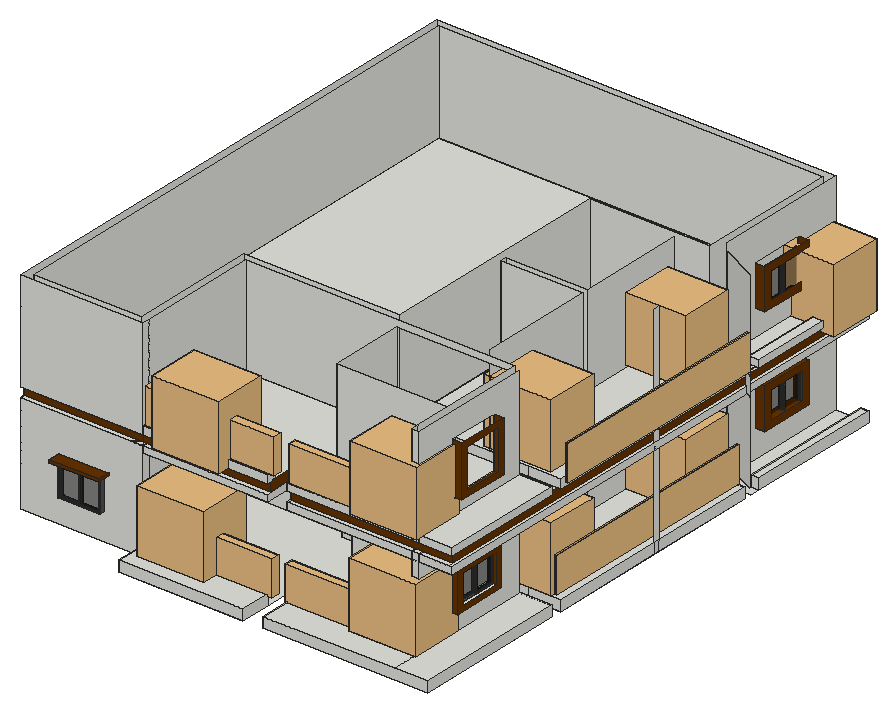
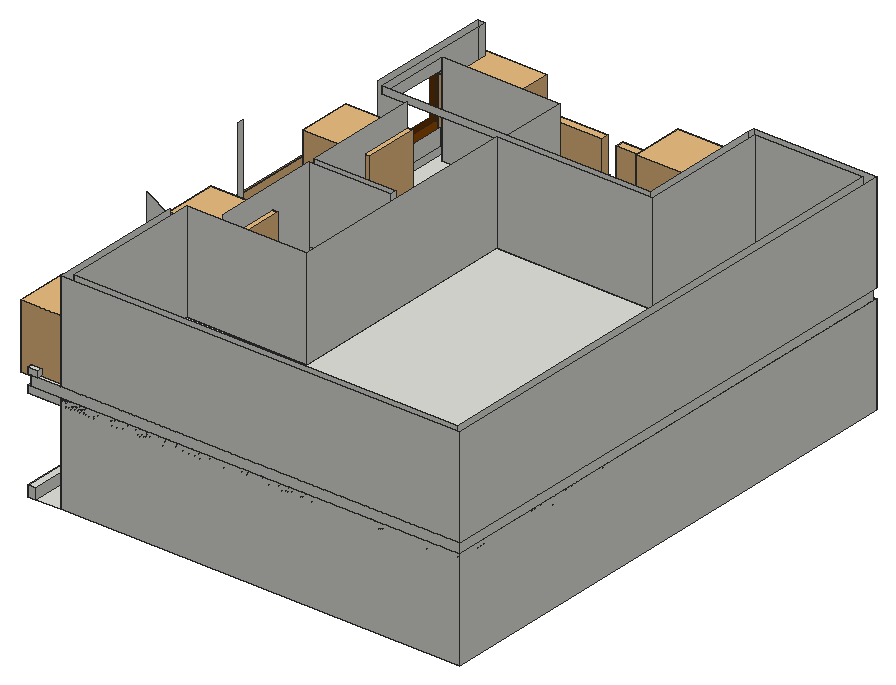
# SketchUp Ruby script. Lengths in inches.
U = 1.inch
M = Sketchup.active_model
def pt(a) = Geom::Point3d.new(a.map { |v| v * U })
def face(e, loops, mat)
  f = e.add_face(loops[0].map { |a| pt(a) })
  loops[1..].each { |l| e.add_face(l.map { |a| pt(a) }).erase! }
  f.material = f.back_material = mat if mat
  f
end
# faces: each face lists its corners as indices into pts; further lists are holes
def faces(e, pts, list, mat = nil) = list.each { |f| face(e, (f[0].is_a?(Array) ? f : [f]).map { |l| l.map { |i| pts[i] } }, mat) }
# xy, xz, yz: faces in a plane at the given z, y or x. An outline is a flat list of corners, or four numbers for a rectangle; further outlines are holes
def ring(l) = l.size == 4 ? [[l[0], l[1]], [l[2], l[1]], [l[2], l[3]], [l[0], l[3]]] : l.each_slice(2).to_a
def flat(e, list, mat, &to3) = list.each { |f| face(e, (f[0].is_a?(Array) ? f : [f]).map { |l| ring(l).map { |u, v| to3.(u, v) } }, mat) }
def xy(e, z, list, mat = nil) = flat(e, list, mat) { |x, y| [x, y, z] }
def xz(e, y, list, mat = nil) = flat(e, list, mat) { |x, z| [x, y, z] }
def yz(e, x, list, mat = nil) = flat(e, list, mat) { |y, z| [x, y, z] }
def lines(e, pts, list) = list.each { |a, b| e.add_line(pt(pts[a]), pt(pts[b])) }
# prism: a flat outline (further loops are holes) pulled along v
def prism(e, loops, v, mat = nil)
  f = face(e, loops, mat); d = Geom::Vector3d.new(v.map { |x| x * U })
  f.pushpull(f.normal.samedirection?(d) ? d.length : -d.length)
end
def box(e, o, s, mat = nil) = prism(e, [[o, [o[0] + s[0], o[1], o[2]], [o[0] + s[0], o[1] + s[1], o[2]], [o[0], o[1] + s[1], o[2]]]], [0, 0, s[2]], mat)
def at(x, y, z, deg = 0) = Geom::Transformation.translation(pt([x, y, z])) * Geom::Transformation.rotation(ORIGIN, Z_AXIS, deg.degrees)
def axes(o, x, y, z) = Geom::Transformation.new([*x, 0, *y, 0, *z, 0, *pt(o).to_a, 1])
def part(name) = M.definitions.add(name)
# library, detail: a bought-in or finely detailed component or shape, given as its bounding box
def library(name, o, s) = part(name).tap { |d| box(d.entities, o, s) }
def detail(e, o, s) = box(e.add_group.entities, o, s)
def put(e, d, t, mat = nil) = e.add_instance(d, t).tap { |i| i.material = mat if mat }
def group(e, t, mat = nil) = e.add_group.tap { |g| g.transformation = t; g.material = mat if mat }.entities
root = M.entities
M.materials.add("Glass_Tinted_Gray").color = [0, 0, 0]
M.materials["Glass_Tinted_Gray"].alpha = 0.125
M.materials.add("[0135_DarkGray]").color = [81, 81, 81]
M.materials.add("[Color C08]").color = [102, 51, 0]
M.materials.add("[Mirror 02]").color = [229, 229, 229]
M.materials.add("[Terrazzo Light Blue]").color = [196, 214, 227]
c1 = library("Round Planter with Plant",[-35.48,-39.77,0],[80.62,63.55,77.875])
c2 = library("Wagner Glass Railing",[9.08,102.375,1.53],[2.51,145.5,42.05])
c3 = part("PENTEK_RP Fineline 50S_Sliding_DoorCase_E1")
box(c3.entities,[0,0,0],[1.51,3.66,99.27],"[0135_DarkGray]")
c4 = part("PENTEK_RP Fineline 50S_SlidingDooe_Case_E2")
box(c4.entities,[0,0,0],[96.25,3.66,1.51],"[0135_DarkGray]")
c5 = part("pentek_RP Fineline 50S_SlidingDoor_Case")
put(c5.entities,c3,at(97.76,0,0))
put(c5.entities,c4,at(1.51,0,0))
put(c5.entities,c3,at(0,0,0))
put(c5.entities,c4,at(1.51,0,97.76))
c6 = part("PENTEK_RP Fineline 50S_SlidingDoor_GlazingBead_2")
box(c6.entities,[0,0,0],[0.56,0.59,94.39],"[0135_DarkGray]")
c7 = part("PENTEK_RP Fineline 50S_SlidingDoor_Glass")
box(c7.entities,[0,0,0],[46.58,0.16,94.39],"Glass_Tinted_Gray")
c8 = part("PENTEK_RP Fineline 50S_SlidingDoor_GlazingBead")
box(c8.entities,[0,0,0],[45.47,0.59,0.56],"[0135_DarkGray]")
c9 = part("PENTEK_RP Fineline 50S_SlidingDoor_Leaf_E1")
xy(c9.entities,0,[[0,0,0.93,1.97],[0.93,1.57,1.49,1.97]],"[0135_DarkGray]")
xy(c9.entities,96.25,[[0,0,0.93,0,0.93,1.57,1.49,1.57,1.49,1.97,0,1.97]],"[0135_DarkGray]")
xz(c9.entities,0,[[0,0,0.93,96.25]],"[0135_DarkGray]")
xz(c9.entities,1.57,[[0.93,0,1.49,95.32],[0.93,95.32,1.49,96.25]],"[0135_DarkGray]")
xz(c9.entities,1.97,[[0,0,1.49,96.25]],"[0135_DarkGray]")
yz(c9.entities,0,[[0,0,1.97,96.25]],"[0135_DarkGray]")
yz(c9.entities,0.93,[[0,0,1.57,0.93],[0,0.93,1.57,95.32],[0,95.32,1.57,96.25]],"[0135_DarkGray]")
yz(c9.entities,1.49,[[1.57,0,1.97,95.32],[1.57,95.32,1.97,96.25]],"[0135_DarkGray]")
c10 = part("PENTEK_RP Fineline 50S_SlidingDoor_Leaf_E2")
xy(c10.entities,0,[[0,0,0,1.57,0.56,1.57,0.56,1.97,46.02,1.97,46.02,1.57,46.58,1.57,46.58,0]],"[0135_DarkGray]")
xy(c10.entities,0.93,[[0,0,46.58,1.57]],"[0135_DarkGray]")
xy(c10.entities,1.49,[[0.56,1.57,46.02,1.97]],"[0135_DarkGray]")
xz(c10.entities,0,[[0,0,46.58,0.93]],"[0135_DarkGray]")
xz(c10.entities,1.57,[[0,0,0.56,0.93],[46.02,0,46.58,0.93],[0.56,0.93,46.02,1.49]],"[0135_DarkGray]")
xz(c10.entities,1.97,[[0.56,0,46.02,1.49]],"[0135_DarkGray]")
yz(c10.entities,0,[[0,0,1.57,0.93]],"[0135_DarkGray]")
yz(c10.entities,0.56,[[1.57,0,1.97,0.93],[1.57,0.93,1.97,1.49]],"[0135_DarkGray]")
yz(c10.entities,46.02,[[1.57,0,1.97,0.93],[1.57,0.93,1.97,1.49]],"[0135_DarkGray]")
yz(c10.entities,46.58,[[0,0,1.57,0.93]],"[0135_DarkGray]")
c11 = part("PENTEK_RP Fineline S_SlidingDoor_Leaf1")
put(c11.entities,c6,at(0.93,0,0.93))
put(c11.entities,c6,at(46.96,0,0.93))
put(c11.entities,c7,at(1.49,1.42,0.93))
put(c11.entities,c8,at(1.49,0,0.93))
put(c11.entities,c7,at(1.49,0.59,0.93),"[Terrazzo Light Blue]")
put(c11.entities,c9,at(0,0,0))
put(c11.entities,c9,axes([48.44,0,0],[-1,0,0],[0,1,0],[0,0,1]))
put(c11.entities,c10,axes([0.93,0,96.25],[1,0,0],[0,1,0],[0,0,-1]))
put(c11.entities,c10,at(0.93,0,0))
put(c11.entities,c8,at(1.49,0,94.77))
c12 = part("PENTEK_RP Fineline 50S_SlidingDoor_Leaf2")
put(c12.entities,c7,at(1.49,1.42,0.93))
put(c12.entities,c8,at(1.49,0,94.77))
put(c12.entities,c6,at(46.96,0,0.93))
put(c12.entities,c7,at(1.49,0.59,0.93),"[Mirror 02]")
put(c12.entities,c6,at(0.93,0,0.93))
put(c12.entities,c9,at(0,0,0))
put(c12.entities,c9,axes([48.44,0,0],[-1,0,0],[0,1,0],[0,0,1]))
put(c12.entities,c8,at(1.49,0,0.93))
put(c12.entities,c10,axes([0.93,0,96.25],[1,0,0],[0,1,0],[0,0,-1]))
put(c12.entities,c10,at(0.93,0,0))
c13 = part("PENTEK - Slimmest Steel Sliding Door / Window\#1")
put(c13.entities,c5,at(0,-1.88,-0.09))
put(c13.entities,c11,at(1.51,-2.27,1.42))
put(c13.entities,c12,at(49.32,-0.3,1.42))
c14 = part("Group\#9")
box(c14.entities,[0,0,0],[60.1875,3.0625,15.3125])
xy(root,264,[[200.56,155.07,350.31,191.22],[374.31,155.07,532.37,191.22],[532.37,155.07,562.5625,155.07,562.5625,162,572.25,162,572.25,341.375,533.0625,341.375,533.0625,191.22,532.37,191.22],[562.5625,155.07,572.25,162],[[53.0625,191.22,200.56,191.22,200.56,346.01,322.375,346.01,322.375,338.57,390.45,338.57,390.45,267.82,524.0625,267.82,524.0625,191.22,532.37,191.22,532.37,341.375,533.0625,341.375,533.0625,355.01,388.3125,355.01,388.3125,631.35,533.0625,631.35,533.0625,818.16,53.0625,818.16],[62.0625,200.22,62.0625,809.84,524.0625,809.84,524.0625,640.35,379.3125,640.35,379.3125,355.01,191.56,355.01,191.56,200.22]],
  [200.56,191.22,350.31,191.22,350.31,232.22,374.31,232.22,374.31,191.22,524.0625,191.22,524.0625,267.82,390.45,267.82,390.45,338.57,322.375,338.57,322.375,346.01,200.56,346.01],[532.37,191.22,533.0625,341.375],[62.0625,200.22,191.56,200.22,191.56,355.01,379.3125,355.01,379.3125,640.35,524.0625,640.35,524.0625,809.84,62.0625,809.84],[388.3125,355.01,572.25,631.35],[533.0625,641.54,572.25,641.54,572.25,653.47,562.82,653.47,562.82,818.16,533.0625,818.16]])
xy(root,276.5625,[[200.56,155.07,350.31,191.22],[374.31,155.07,532.37,191.22],[532.37,155.07,572.25,341.375],[388.3125,355.01,486.8125,495.28],[486.8125,355.01,572.25,355.01,572.25,631.35,486.8125,631.35,486.8125,502.74,388.3125,502.74,388.3125,495.28,486.8125,495.28],
  [388.3125,502.74,486.8125,631.35],[562.82,653.47,572.25,818.16]])
xy(root,298.54,[[533.0625,696.28,545.1875,761.47]],"[Color C08]")
xy(root,303.83,[[533.0625,234.02,545.1875,299.52]],"[Color C08]")
xy(root,306.6,[[533.0625,704.34,545.1875,753.42]],"[Color C08]")
xy(root,310.91,[[533.0625,241.1,545.1875,292.4375]])
xy(root,339.68,[[533.0625,704.34,545.1875,753.42]])
xy(root,346.18,[[533.0625,241.1,545.1875,292.4375]],"[Color C08]")
xy(root,347.73,[[533.0625,696.28,545.1875,761.47]],"[Color C08]")
xy(root,353.26,[[533.0625,234.02,545.1875,299.52]],"[Color C08]")
xy(root,375.8125,[[390.45,267.82,524.0625,267.82,524.0625,346.01,412.14,346.01,412.14,338.57,390.45,338.57],[322.375,338.57,412.14,346.01]])
xy(root,384,[[[53.0625,191.22,200.56,191.22,200.56,346.01,524.0625,346.01,524.0625,191.22,533.0625,191.22,533.0625,355.01,486.8125,355.01,486.8125,495.28,388.3125,495.28,388.3125,502.74,486.8125,502.74,486.8125,631.35,533.0625,631.35,533.0625,818.16,53.0625,818.16],[62.0625,200.22,62.0625,809.84,524.0625,809.84,524.0625,640.35,379.3125,640.35,379.3125,355.01,191.56,355.01,191.56,200.22]]])
xy(root,396,[[[53.0625,191.22,200.56,191.22,200.56,346.01,381.78,346.01,381.78,256.07,524.0625,256.07,524.0625,191.22,532.82,191.22,532.82,341.375,533.0625,341.375,533.0625,355.01,388.3125,355.01,388.3125,631.35,533.0625,631.35,533.0625,818.16,53.0625,818.16],[62.0625,200.22,62.0625,809.84,524.0625,809.84,524.0625,640.35,379.3125,640.35,379.3125,355.01,191.56,355.01,191.56,200.22]],[532.82,191.22,533.0625,341.375],[62.0625,200.22,191.56,200.22,191.56,355.01,379.3125,355.01,379.3125,640.35,524.0625,640.35,524.0625,809.84,62.0625,809.84],[374.31,200.22,524.0625,200.22,524.0625,256.07,381.78,256.07,381.78,346.01,200.56,346.01,200.56,202.86,350.31,202.86,350.31,232.22,374.31,232.22],[388.3125,355.01,572.25,631.35],
  [533.0625,641.54,572.25,641.54,572.25,653.47,559.99,653.47,559.99,818.16,533.0625,818.16]])
xy(root,404.1875,[[532.82,191.22,572.25,341.375],[559.99,653.47,572.25,818.16]])
xy(root,405.4375,[[200.56,191.22,350.31,202.86],[374.31,191.22,524.0625,200.22]])
xy(root,407.125,[[388.3125,355.01,486.8125,495.28],[486.8125,355.01,572.25,355.01,572.25,631.35,486.8125,631.35,486.8125,502.74,388.3125,502.74,388.3125,495.28,486.8125,495.28],[388.3125,502.74,486.8125,631.35]])
xy(root,424.41,[[533.0625,240.75,545.1875,302.81]],"[Color C08]")
xy(root,427.36,[[533.0625,696.28,545.1875,761.47]],"[Color C08]")
xz(root,155.07,[[200.56,264,350.31,276.5625],[374.31,264,572.25,276.5625]])
xz(root,191.22,[[53.0625,264,200.56,384],[200.56,264,350.31,276.5625],[374.31,264,524.0625,276.5625],[524.0625,264,532.37,276.5625],[532.37,264,533.0625,264,533.0625,384,524.0625,384,524.0625,276.5625,532.37,276.5625],
  [53.0625,396,200.56,516],[200.56,396,350.31,405.4375],[374.31,396,524.0625,405.4375],[524.0625,396,532.82,396,532.82,404.1875,533.0625,404.1875,533.0625,516,524.0625,516],[532.82,396,533.0625,404.1875],
  [533.0625,396,572.25,404.1875]])
xz(root,200.22,[[62.0625,264,191.56,384],[62.0625,396,191.56,516],[374.31,396,524.0625,405.4375]])
xz(root,202.86,[[200.56,396,350.31,405.4375]])
xz(root,234.02,[[533.0625,303.83,545.1875,353.26]],"[Color C08]")
xz(root,240.75,[[533.0625,424.41,545.1875,486.47]],"[Color C08]")
xz(root,241.1,[[533.0625,310.91,545.1875,346.18]],"[Color C08]")
xz(root,256.07,[[381.78,396,524.0625,507.8125]])
xz(root,267.82,[[390.45,264,524.0625,375.8125]])
xz(root,292.4375,[[533.0625,310.91,545.1875,346.18]],"[Color C08]")
xz(root,299.52,[[533.0625,303.83,545.1875,353.26]],"[Color C08]")
xz(root,302.81,[[533.0625,424.41,545.1875,486.47]],"[Color C08]")
xz(root,338.57,[[322.375,264,390.45,375.8125]])
xz(root,341.375,[[532.37,264,533.0625,276.5625],[533.0625,264,572.25,276.5625],[532.82,396,533.0625,404.1875],[533.0625,396,572.25,404.1875]])
xz(root,346.01,[[200.56,264,322.375,264,322.375,375.8125,524.0625,375.8125,524.0625,384,200.56,384],[200.56,396,381.78,396,381.78,507.8125,524.0625,507.8125,524.0625,516,200.56,516]])
xz(root,355.01,[[191.56,264,379.3125,384],[388.3125,264,533.0625,276.5625],[533.0625,264,572.25,276.5625],[191.56,396,379.3125,516],[388.3125,396,533.0625,407.125],
  [533.0625,396,572.25,407.125]])
xz(root,495.28,[[388.3125,276.5625,486.8125,294.1875],[388.3125,294.1875,486.8125,384],[388.3125,407.125,486.8125,424.625],[388.3125,424.625,486.8125,516]])
xz(root,502.74,[[388.3125,276.5625,486.8125,294.1875],[388.3125,294.1875,486.8125,384],[388.3125,407.125,486.8125,424.625],[388.3125,424.625,486.8125,516]])
xz(root,631.35,[[388.3125,264,533.0625,276.5625],[533.0625,264,572.25,276.5625],[388.3125,396,533.0625,407.125],[533.0625,396,572.25,407.125]])
xz(root,640.35,[[379.3125,264,524.0625,384],[379.3125,396,524.0625,516]])
xz(root,653.47,[[562.82,264,572.25,276.5625],[559.99,396,572.25,404.1875]])
xz(root,696.28,[[533.0625,298.54,545.1875,347.73],[533.0625,427.36,545.1875,476.54]],"[Color C08]")
xz(root,704.34,[[533.0625,306.6,545.1875,339.68]],"[Color C08]")
xz(root,753.42,[[533.0625,306.6,545.1875,339.68]],"[Color C08]")
xz(root,761.47,[[533.0625,298.54,545.1875,347.73],[533.0625,427.36,545.1875,476.54]],"[Color C08]")
xz(root,809.84,[[62.0625,264,524.0625,384],[62.0625,396,524.0625,516]])
xz(root,818.16,[[53.0625,264,533.0625,384],[562.82,264,572.25,276.5625],[53.0625,396,533.0625,516],[559.99,396,572.25,404.1875]])
yz(root,53.0625,[[191.22,264,818.16,384],[191.22,396,818.16,516]])
yz(root,62.0625,[[200.22,264,809.84,384],[200.22,396,809.84,516]])
yz(root,191.56,[[200.22,264,355.01,384],[200.22,396,355.01,516]])
yz(root,200.56,[[155.07,264,191.22,276.5625],[191.22,264,200.22,384],[200.22,264,346.01,384],[191.22,396,200.22,405.4375],[200.22,396,202.86,405.4375],
  [202.86,396,346.01,396,346.01,516,200.22,516,200.22,405.4375,202.86,405.4375],[191.22,405.4375,200.22,516]])
yz(root,322.375,[[338.57,264,346.01,375.8125]])
yz(root,350.31,[[155.07,264,191.22,276.5625],[191.22,396,202.86,405.4375]])
yz(root,374.31,[[155.07,264,191.22,276.5625],[191.22,396,200.22,405.4375]])
yz(root,379.3125,[[355.01,264,640.35,384],[355.01,396,640.35,516]])
yz(root,381.78,[[256.07,396,346.01,507.8125]])
yz(root,388.3125,[[355.01,264,495.28,276.5625],[495.28,264,502.74,276.5625],[502.74,264,631.35,276.5625],[495.28,276.5625,502.74,294.1875],[495.28,294.1875,502.74,384],
  [495.28,384,502.74,396],[355.01,396,495.28,407.125],[495.28,396,502.74,407.125],[502.74,396,631.35,407.125],[495.28,407.125,502.74,424.625],
  [495.28,424.625,502.74,516]])
yz(root,390.45,[[267.82,264,338.57,375.8125]])
yz(root,486.8125,[[355.01,276.5625,495.28,384],[502.74,276.5625,631.35,384],[355.01,407.125,495.28,516],[502.74,407.125,631.35,516]])
yz(root,524.0625,[[191.22,264,200.22,384],[200.22,264,200.22,384,346.01,384,346.01,375.8125,267.82,375.8125,267.82,264],[640.35,264,809.84,384],[191.22,396,200.22,405.4375],[200.22,396,200.22,516,346.01,516,346.01,507.8125,256.07,507.8125,256.07,396],
  [640.35,396,809.84,516],[191.22,405.4375,200.22,516]])
yz(root,532.37,[[191.22,264,341.375,276.5625]])
yz(root,532.82,[[191.22,396,341.375,404.1875]])
yz(root,533.0625,[[[191.22,264,341.375,384],[234.02,303.83,299.52,353.26]],[[653.47,264,818.16,384],[696.28,298.54,761.47,347.73]],[704.34,306.6,753.42,339.68],[241.1,310.91,292.4375,346.18],[341.375,384,355.01,396],
  [631.35,384,653.47,396],[[191.22,396,341.375,516],[240.75,424.41,302.81,486.47]],[[653.47,396,818.16,516],[696.28,427.36,761.47,476.54]]])
yz(root,545.1875,[[[696.28,298.54,761.47,347.73],[704.34,306.6,753.42,339.68]],[[234.02,303.83,299.52,353.26],[241.1,310.91,292.4375,346.18]],[[240.75,424.41,302.81,486.47],[247.82,431.49,295.73,479.39]],[[696.28,427.36,761.47,476.54],[704.34,435.41,753.42,468.49]]],"[Color C08]")
yz(root,559.99,[[653.47,396,818.16,404.1875]])
yz(root,562.82,[[653.47,264,818.16,276.5625]])
yz(root,572.25,[[155.07,264,341.375,276.5625],[355.01,264,495.28,276.5625],[495.28,264,502.74,276.5625],[502.74,264,631.35,276.5625],[653.47,264,818.16,276.5625],
  [495.28,276.5625,502.74,396],[191.22,396,341.375,404.1875],[355.01,396,495.28,407.125],[495.28,396,502.74,407.125],[502.74,396,631.35,407.125],
  [653.47,396,818.16,404.1875],[495.28,407.125,502.74,528]])
p = [[578.3125,631.35,375.8125],[533.0625,653.47,375.8125],[533.0625,653.47,277.47],[578.3125,631.35,277.47],[578.3125,631.35,398.63],[533.0625,653.47,398.63],
  [533.0625,653.47,396],[533.0625,653.47,384],[578.3125,631.35,507.8125],[533.0625,653.47,507.8125],[200.56,191.22,396],[200.56,191.22,384]]
faces(root,p,[[0,1,2,3],[4,5,6,7,1,0],[5,4,8,9]])
lines(root,p,[[10,11]])
put(root,c1,at(243.82,211.68,273.97))
put(root,c2,axes([90.83,155.01,273.31],[0,3.9,0],[1.07184,0,0],[0,0,1]))
put(root,c2,axes([262.52,155.01,273.31],[0,3.9,0],[1.07184,0,0],[0,0,1]))
put(root,c1,at(515.72,394.78,277.14))
put(root,c1,at(515.28,598.17,277.7))
put(root,c2,axes([554.35,165.24,276.5625],[1,0,0],[0,1.88042,0],[0,0,1]))
put(root,c1,at(492.57,220.35,279.59))
put(root,c13,axes([153.96,188.68,296.18],[-0.51717,0,0],[0,1.4209,0],[0,0,0.41395]))
put(root,c13,axes([538.58,754.625,299.68],[0,-0.51717,0],[-1.4209,0,0],[0,0,0.41395]))
put(root,c13,axes([538.58,292.4375,310.57],[0,-0.51717,0],[-1.4209,0,0],[0,0,0.41395]))
put(root,c14,axes([99.21,191.22,337.07],[1,0,0],[0,0,1],[0,-1,0]),"[Color C08]")
g1 = group(root,at(53.0625,818.16,384))
xy(g1,-8.1875,[[0,-626.9375,0,0,519.1875,0,519.1875,-626.9375,321.25,-626.9375,321.25,-586.6875,297.25,-586.6875,297.25,-626.9375]],"[Color C08]")
xy(g1,0,[[0,-626.9375,297.25,-621.1875],[321.25,-626.9375,515.4375,-621.1875],[515.4375,-626.9375,519.1875,0],[0,-621.1875,297.25,-621.1875,297.25,-586.6875,321.25,-586.6875,321.25,-621.1875,515.4375,-621.1875,515.4375,0,0,0]])
xz(g1,-626.9375,[[0,-8.1875,297.25,0],[321.25,-8.1875,519.1875,0]])
xz(g1,-621.1875,[[0,0,297.25,12],[321.25,0,515.4375,12]],"[Color C08]")
xz(g1,-586.6875,[[297.25,-8.1875,321.25,0]])
xz(g1,-586.6875,[[297.25,0,321.25,12]],"[Color C08]")
xz(g1,0,[[0,-8.1875,519.1875,0],[0,0,515.4375,12]])
yz(g1,0,[[-626.9375,-8.1875,0,0],[-621.1875,0,0,12]])
yz(g1,297.25,[[-626.9375,-8.1875,-586.6875,0]])
yz(g1,297.25,[[-621.1875,0,-586.6875,12]],"[Color C08]")
yz(g1,321.25,[[-626.9375,-8.1875,-586.6875,0]])
yz(g1,321.25,[[-621.1875,0,-586.6875,12]],"[Color C08]")
yz(g1,515.4375,[[-621.1875,0,0,12]],"[Color C08]")
yz(g1,519.1875,[[-626.9375,-8.1875,0,0]])
put(root,c1,at(540.42,789.45,391.58))
put(root,c1,at(257.97,217.07,395.56))
put(root,c2,axes([566.72,165.24,401.65],[1,0,0],[0,1.88042,0],[0,0,1]))
put(root,c1,at(490.68,223.38,403.64))
put(root,c2,axes([271.66,155.82,403.89],[0,3.9,0],[1.01825,0,0],[0,0,1]))
put(root,c2,axes([90.56,158.16,404.12],[0,3.9,0],[1.07184,0,0],[0,0,1]))
put(root,c1,at(515.72,394.78,410.39))
put(root,c1,at(515.28,598.17,410.95))
put(root,c13,axes([538.58,754.625,428.49],[0,-0.51717,0],[-1.4209,0,0],[0,0,0.41395]))
